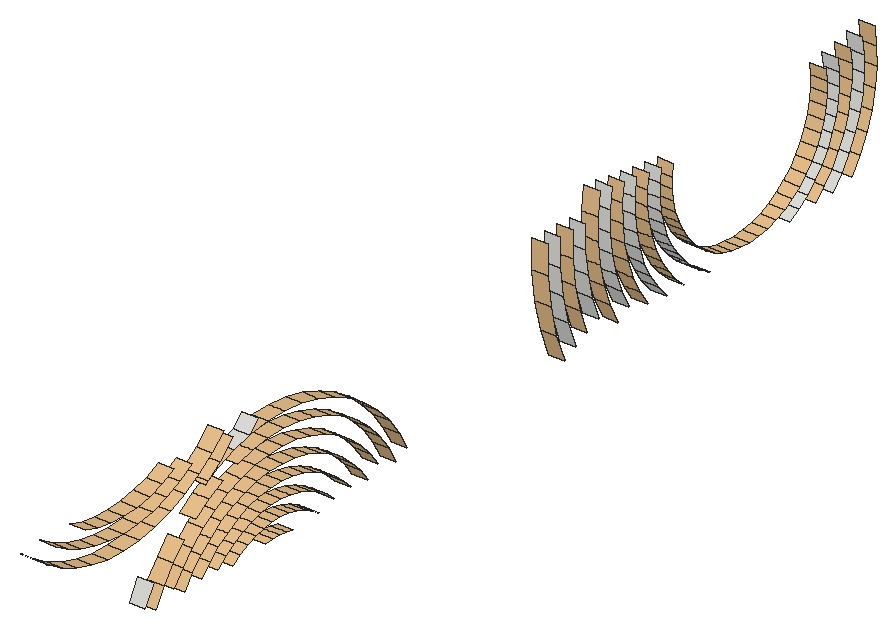
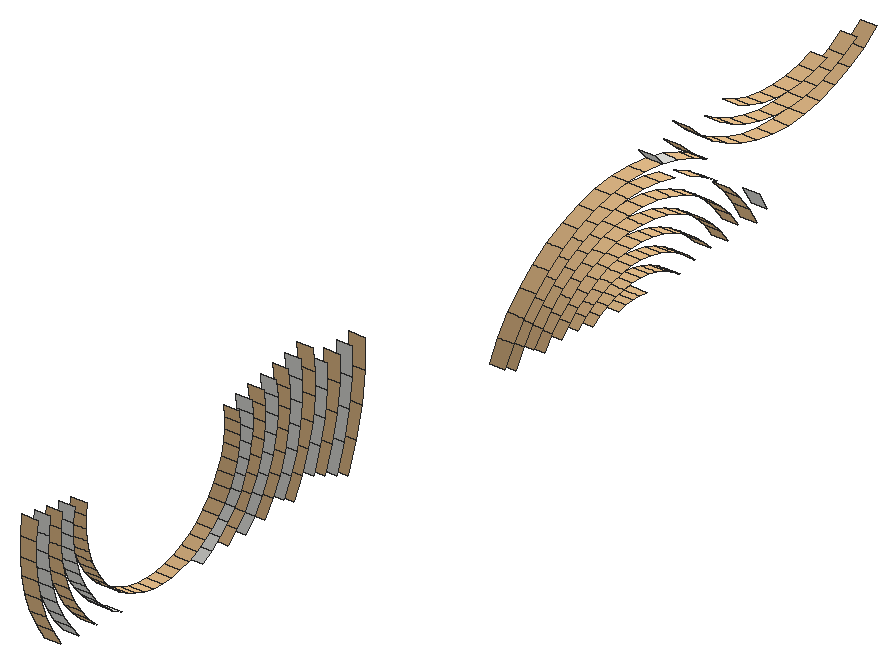
# SketchUp Ruby script. Lengths in inches.
U = 1.inch
M = Sketchup.active_model
def pt(a) = Geom::Point3d.new(a.map { |v| v * U })
def face(e, loops, mat)
  f = e.add_face(loops[0].map { |a| pt(a) })
  loops[1..].each { |l| e.add_face(l.map { |a| pt(a) }).erase! }
  f.material = f.back_material = mat if mat
  f
end
# faces: each face lists its corners as indices into pts; further lists are holes
def faces(e, pts, list, mat = nil) = list.each { |f| face(e, (f[0].is_a?(Array) ? f : [f]).map { |l| l.map { |i| pts[i] } }, mat) }
# xy, xz, yz: faces in a plane at the given z, y or x. An outline is a flat list of corners, or four numbers for a rectangle; further outlines are holes
def ring(l) = l.size == 4 ? [[l[0], l[1]], [l[2], l[1]], [l[2], l[3]], [l[0], l[3]]] : l.each_slice(2).to_a
def flat(e, list, mat, &to3) = list.each { |f| face(e, (f[0].is_a?(Array) ? f : [f]).map { |l| ring(l).map { |u, v| to3.(u, v) } }, mat) }
def xy(e, z, list, mat = nil) = flat(e, list, mat) { |x, y| [x, y, z] }
def xz(e, y, list, mat = nil) = flat(e, list, mat) { |x, z| [x, y, z] }
def yz(e, x, list, mat = nil) = flat(e, list, mat) { |y, z| [x, y, z] }
def lines(e, pts, list) = list.each { |a, b| e.add_line(pt(pts[a]), pt(pts[b])) }
# prism: a flat outline (further loops are holes) pulled along v
def prism(e, loops, v, mat = nil)
  f = face(e, loops, mat); d = Geom::Vector3d.new(v.map { |x| x * U })
  f.pushpull(f.normal.samedirection?(d) ? d.length : -d.length)
end
def box(e, o, s, mat = nil) = prism(e, [[o, [o[0] + s[0], o[1], o[2]], [o[0] + s[0], o[1] + s[1], o[2]], [o[0], o[1] + s[1], o[2]]]], [0, 0, s[2]], mat)
def at(x, y, z, deg = 0) = Geom::Transformation.translation(pt([x, y, z])) * Geom::Transformation.rotation(ORIGIN, Z_AXIS, deg.degrees)
def axes(o, x, y, z) = Geom::Transformation.new([*x, 0, *y, 0, *z, 0, *pt(o).to_a, 1])
def part(name) = M.definitions.add(name)
# library, detail: a bought-in or finely detailed component or shape, given as its bounding box
def library(name, o, s) = part(name).tap { |d| box(d.entities, o, s) }
def detail(e, o, s) = box(e.add_group.entities, o, s)
def put(e, d, t, mat = nil) = e.add_instance(d, t).tap { |i| i.material = mat if mat }
def group(e, t, mat = nil) = e.add_group.tap { |g| g.transformation = t; g.material = mat if mat }.entities
root = M.entities
M.materials.add("images").color = [235, 194, 141]
xy(root,18.6875,[[183.82,93.83,185.82,94.95]],"images")
xy(root,20.69,[[183.82,93.71,185.82,95.07]],"images")
xy(root,22.68,[[183.82,93.6,185.82,95.18]],"images")
xy(root,24.68,[[183.82,93.48,185.82,95.3]],"images")
xy(root,26.68,[[183.82,93.36,185.82,95.41]],"images")
xy(root,28.67,[[183.82,93.25,185.82,95.53]],"images")
xy(root,30.67,[[183.82,93.13,185.82,95.65]],"images")
xy(root,32.61,[[183.82,93.02,185.82,95.76]],"images")
xz(root,182.85,[[183.82,30.9375,185.82,32.39]],"images")
p = [[183.82,96.0625,18.56],[183.82,97.15,18.3],[185.82,97.15,18.3],[185.82,96.0625,18.56],[183.82,88.58,19.15],[183.82,87.45,18.4],
  [185.82,87.45,18.4],[185.82,88.58,19.15],[183.82,101.33,18.4],[183.82,100.2,19.15],[185.82,100.2,19.15],[185.82,101.33,18.4],
  [183.82,92.72,18.56],[183.82,93.83,18.6875],[185.82,93.83,18.6875],[185.82,92.72,18.56],[183.82,94.95,18.6875],[185.82,94.95,18.6875],
  [183.82,139.41,22.1],[183.82,140.73,18.57],[185.82,140.73,18.57],[185.82,139.41,22.1],[183.82,164.03,18.65],[183.82,162.57,19.48],
  [185.82,162.57,19.48],[185.82,164.03,18.65],[183.82,178.4375,19.57],[183.82,176.99,18.73],[185.82,176.99,18.73],[185.82,178.4375,19.57],
  [183.82,75.06,18.79],[183.82,76.32,20.96],[185.82,76.32,20.96],[185.82,75.06,18.79],[183.82,79.66,18.77],[183.82,80.89,20.41],
  [185.82,80.89,20.41],[185.82,79.66,18.77],[183.82,107.89,20.41],[183.82,109.12,18.77],[185.82,109.12,18.77],[185.82,107.89,20.41],
  [183.82,112.46,20.96],[183.82,113.71,18.79],[185.82,113.71,18.79],[185.82,112.46,20.96],[183.82,157.1,18.86],[183.82,155.71,20.49],
  [185.82,155.71,20.49],[185.82,157.1,18.86],[183.82,158.54,20.24],[183.82,159.94,18.94],[185.82,159.94,18.94],[185.82,158.54,20.24],
  [183.82,85.04,18.99],[183.82,86.25,20.01],[185.82,86.25,20.01],[185.82,85.04,18.99],[183.82,102.53,20.01],[183.82,103.74,18.99],
  [185.82,103.74,18.99],[185.82,102.53,20.01],[183.82,185.29,20.67],[183.82,183.92,19.02],[185.82,183.92,19.02],[185.82,185.29,20.67],
  [183.82,83.67,20.45],[183.82,82.42,19.125],[185.82,82.42,19.125],[185.82,83.67,20.45],[183.82,89.79,19.75],[185.82,89.79,19.75],
  [183.82,98.99,19.75],[185.82,98.99,19.75],[183.82,106.36,19.125],[183.82,105.11,20.45],[185.82,105.11,20.45],[185.82,106.36,19.125],
  [183.82,181.07,19.06],[183.82,182.46,20.38],[185.82,182.46,20.38],[185.82,181.07,19.06],[183.82,148.05,21.78],[183.82,149.34,19.25],
  [185.82,149.34,19.25],[185.82,148.05,21.78],[183.82,167.64,19.47],[183.82,169.0625,19.23],[185.82,169.0625,19.23],[185.82,167.64,19.47],
  [183.82,170.51,19.15],[185.82,170.51,19.15],[183.82,171.95,19.24],[185.82,171.95,19.24],[183.82,173.375,19.5],[185.82,173.375,19.5],
  [183.82,152.8,21.27],[183.82,154.11,19.29],[185.82,154.11,19.29],[185.82,152.8,21.27],[183.82,142.56,19.37],[183.82,141.33,22.6875],
  [185.82,141.33,22.6875],[185.82,142.56,19.37],[183.82,161.22,20.47],[185.82,161.22,20.47],[183.82,166.25,19.875],[185.82,166.25,19.875],
  [183.82,174.76,19.93],[185.82,174.76,19.93],[183.82,186.9,19.48],[183.82,188.19,21.48],[185.82,188.19,21.48],[185.82,186.9,19.48],
  [183.82,179.78,20.58],[185.82,179.78,20.58],[183.82,74.7,22.03],[183.82,73.33,19.66],[185.82,73.33,19.66],[185.82,74.7,22.03],
  [183.82,115.45,19.66],[183.82,114.08,22.03],[185.82,114.08,22.03],[185.82,115.45,19.66],[183.82,91.06,20.22],[185.82,91.06,20.22],
  [183.82,97.72,20.22],[185.82,97.72,20.22],[183.82,79.36,21.69],[183.82,77.99,19.86],[185.82,77.99,19.86],[185.82,79.36,21.69],
  [183.82,110.79,19.86],[183.82,109.42,21.69],[185.82,109.42,21.69],[185.82,110.79,19.86],[183.82,164.92,20.44],[185.82,164.92,20.44],
  [183.82,176.08,20.51],[185.82,176.08,20.51],[183.82,87.58,20.88],[185.82,87.58,20.88],[183.82,101.2,20.88],[185.82,101.2,20.88],
  [183.82,92.37,20.53],[185.82,92.37,20.53],[183.82,96.41,20.53],[185.82,96.41,20.53],[183.82,143.24,23.27],[183.82,144.39,20.17],
  [185.82,144.39,20.17],[185.82,143.24,23.27],[183.82,157.31,21.7],[185.82,157.31,21.7],[183.82,151.07,20.26],[183.82,149.88,22.58],
  [185.82,149.88,22.58],[185.82,151.07,20.26],[183.82,82.29,21.9],[185.82,82.29,21.9],[183.82,85.06,21.61],[185.82,85.06,21.61],
  [183.82,103.72,21.61],[185.82,103.72,21.61],[183.82,106.48,21.9],[185.82,106.48,21.9],[183.82,163.66,21.16],[185.82,163.66,21.16],
  [183.82,183.68,21.85],[185.82,183.68,21.85],[183.82,93.71,20.69],[185.82,93.71,20.69],[183.82,95.07,20.69],[185.82,95.07,20.69],
  [183.82,154.52,22.28],[185.82,154.52,22.28],[183.82,159.99,21.62],[185.82,159.99,21.62],[183.82,177.33,21.24],[185.82,177.33,21.24],
  [183.82,180.99,21.74],[185.82,180.99,21.74],[183.82,186.46,22.46],[185.82,186.46,22.46],[183.82,88.99,21.59],[185.82,88.99,21.59],
  [183.82,99.79,21.59],[185.82,99.79,21.59],[183.82,77.82,22.98],[185.82,77.82,22.98],[183.82,110.96,22.98],[185.82,110.96,22.98],
  [183.82,146.22,20.97],[183.82,145.15,23.86],[185.82,145.15,23.86],[185.82,146.22,20.97],[183.82,162.5,22.01],[185.82,162.5,22.01],
  [183.82,178.49,22.11],[185.82,178.49,22.11],[183.82,151.72,23.38],[185.82,151.72,23.38],[183.82,189.25,23.61],[185.82,189.25,23.61],
  [183.82,86.58,22.61],[185.82,86.58,22.61],[183.82,90.48,22.13],[185.82,90.48,22.13],[183.82,98.3,22.13],[185.82,98.3,22.13],
  [183.82,102.2,22.61],[185.82,102.2,22.61],[183.82,158.9,22.9],[185.82,158.9,22.9],[183.82,80.92,23.35],[185.82,80.92,23.35],
  [183.82,107.86,23.35],[185.82,107.86,23.35],[183.82,156.25,23.29],[185.82,156.25,23.29],[183.82,182.07,23.04],[185.82,182.07,23.04],
  [183.82,147.07,24.44],[185.82,147.07,24.44],[183.82,83.86,23.22],[185.82,83.86,23.22],[183.82,104.91,23.22],[185.82,104.91,23.22],
  [183.82,184.72,23.45],[185.82,184.72,23.45],[183.82,112.44,24.23],[185.82,112.44,24.23],[183.82,161.4375,23],[185.82,161.4375,23],
  [183.82,92.02,22.5],[185.82,92.02,22.5],[183.82,96.76,22.5],[185.82,96.76,22.5],[183.82,138.52,25.77],[185.82,138.52,25.77],
  [183.82,179.53,23.11],[185.82,179.53,23.11],[183.82,153.55,24.1875],[185.82,153.55,24.1875],[183.82,93.6,22.68],[185.82,93.6,22.68],
  [183.82,95.18,22.68],[185.82,95.18,22.68],[183.82,187.41,24.39],[185.82,187.41,24.39],[183.82,88.2,23.43],[185.82,88.2,23.43],
  [183.82,100.58,23.43],[185.82,100.58,23.43],[183.82,148.98,25.03],[185.82,148.98,25.03],[183.82,140.49,26.125],[185.82,140.49,26.125],
  [183.82,157.97,24.3],[185.82,157.97,24.3],[183.82,79.55,24.81],[185.82,79.55,24.81],[183.82,109.23,24.81],[185.82,109.23,24.81],
  [183.82,160.5,24.1],[185.82,160.5,24.1],[183.82,182.98,24.44],[185.82,182.98,24.44],[183.82,180.45,24.22],[185.82,180.45,24.22],
  [183.82,85.58,24.34],[185.82,85.58,24.34],[183.82,103.2,24.34],[185.82,103.2,24.34],[183.82,142.46,26.49],[185.82,142.46,26.49],
  [183.82,155.38,24.99],[185.82,155.38,24.99],[183.82,82.67,24.82],[185.82,82.67,24.82],[183.82,89.91,24.05],[185.82,89.91,24.05],
  [183.82,98.87,24.05],[185.82,98.87,24.05],[183.82,106.11,24.82],[185.82,106.11,24.82],[183.82,150.89,25.61],[185.82,150.89,25.61],
  [183.82,185.57,25.17],[185.82,185.57,25.17],[183.82,190.05,25.84],[185.82,190.05,25.84],[183.82,144.43,26.84],[185.82,144.43,26.84],
  [183.82,91.68,24.47],[185.82,91.68,24.47],[183.82,97.1,24.47],[185.82,97.1,24.47],[183.82,159.7,25.31],[185.82,159.7,25.31],
  [183.82,110.5625,26.22],[185.82,110.5625,26.22],[183.82,152.8,26.2],[185.82,152.8,26.2],[183.82,181.24,25.43],[185.82,181.24,25.43],
  [183.82,87.41,25.26],[185.82,87.41,25.26],[183.82,101.37,25.26],[185.82,101.37,25.26],[183.82,157.21,25.79],[185.82,157.21,25.79],
  [183.82,146.39,27.2],[185.82,146.39,27.2],[183.82,183.72,25.95],[185.82,183.72,25.95],[183.82,188.13,26.41],[185.82,188.13,26.41],
  [183.82,93.48,24.68],[185.82,93.48,24.68],[183.82,95.3,24.68],[185.82,95.3,24.68],[183.82,84.58,26.08],[185.82,84.58,26.08],
  [183.82,104.2,26.08],[185.82,104.2,26.08],[183.82,107.3,26.43],[185.82,107.3,26.43],[183.82,148.36,27.5625],[185.82,148.36,27.5625],
  [183.82,154.72,26.78],[185.82,154.72,26.78],[183.82,186.21,26.97],[185.82,186.21,26.97],[183.82,89.33,25.96],[185.82,89.33,25.96],
  [183.82,99.44,25.96],[185.82,99.44,25.96],[183.82,159.04,26.6],[185.82,159.04,26.6],[183.82,181.88,26.73],[185.82,181.88,26.73],
  [183.82,150.33,27.92],[185.82,150.33,27.92],[183.82,138.0625,29.51],[185.82,138.0625,29.51],[183.82,156.63,27.37],[185.82,156.63,27.37],
  [183.82,190.58,28.16],[185.82,190.58,28.16],[183.82,184.29,27.53],[185.82,184.29,27.53],[183.82,91.33,26.4375],[185.82,91.33,26.4375],
  [183.82,97.45,26.4375],[185.82,97.45,26.4375],[183.82,86.62,27.1],[185.82,86.62,27.1],[183.82,102.16,27.1],[185.82,102.16,27.1],
  [183.82,140.06,29.64],[185.82,140.06,29.64],[183.82,108.46,27.98],[185.82,108.46,27.98],[183.82,152.3,28.28],[185.82,152.3,28.28],
  [183.82,81.48,26.43],[183.82,83.58,27.81],[185.82,83.58,27.81],[185.82,81.48,26.43],[183.82,93.36,26.68],[185.82,93.36,26.68],
  [183.82,95.41,26.68],[185.82,95.41,26.68],[183.82,105.2,27.81],[185.82,105.2,27.81],[183.82,188.61,28.49],[185.82,188.61,28.49],
  [183.82,142.06,29.77],[185.82,142.06,29.77],[183.82,158.54,27.95],[185.82,158.54,27.95],[183.82,182.37,28.09],[185.82,182.37,28.09],
  [183.82,144.05,29.9],[185.82,144.05,29.9],[183.82,154.26,28.64],[185.82,154.26,28.64],[183.82,186.64,28.83],[185.82,186.64,28.83],
  [183.82,88.76,27.88],[185.82,88.76,27.88],[183.82,100.02,27.88],[185.82,100.02,27.88],[183.82,146.05,30.02],[185.82,146.05,30.02],
  [183.82,156.23,29],[185.82,156.23,29],[183.82,184.67,29.17],[185.82,184.67,29.17],[183.82,148.04,30.15],[185.82,148.04,30.15],
  [183.82,67.36,27.94],[183.82,69.91,27.78],[185.82,69.91,27.78],[185.82,67.36,27.94],[183.82,72.47,27.92],[185.82,72.47,27.92],
  [183.82,85.82,28.9375],[185.82,85.82,28.9375],[183.82,102.96,28.9375],[185.82,102.96,28.9375],[183.82,64.84,28.4],[185.82,64.84,28.4],
  [183.82,74.99,28.35],[185.82,74.99,28.35],[183.82,90.98,28.41],[185.82,90.98,28.41],[183.82,97.8,28.41],[185.82,97.8,28.41],
  [183.82,150.04,30.28],[185.82,150.04,30.28],[183.82,106.17,29.49],[185.82,106.17,29.49],[183.82,158.2,29.36],[185.82,158.2,29.36],
  [183.82,182.7,29.5],[185.82,182.7,29.5],[183.82,190.84,30.52],[185.82,190.84,30.52],[183.82,152.03,30.41],[185.82,152.03,30.41],
  [183.82,62.39,29.15],[185.82,62.39,29.15],[183.82,77.44,29.07],[185.82,77.44,29.07],[183.82,93.25,28.67],[185.82,93.25,28.67],
  [183.82,95.53,28.67],[185.82,95.53,28.67],[183.82,188.85,30.625],[185.82,188.85,30.625],[183.82,154.03,30.54],[185.82,154.03,30.54],
  [183.82,186.85,30.73],[185.82,186.85,30.73],[183.82,100.59,29.8],[185.82,100.59,29.8],[183.82,156.03,30.66],[185.82,156.03,30.66],
  [183.82,60.05,30.17],[185.82,60.05,30.17],[183.82,79.8,30.07],[185.82,79.8,30.07],[183.82,184.85,30.83],[185.82,184.85,30.83],
  [183.82,158.02,30.79],[185.82,158.02,30.79],[183.82,103.72,30.72],[185.82,103.72,30.72],[183.82,138.04,33.28],[185.82,138.04,33.28],
  [183.82,182.85,30.9375],[185.82,182.85,30.9375],[183.82,140.04,33.18],[185.82,140.04,33.18],[183.82,83.42,29.9],[183.82,83.11,29.67],
  [185.82,83.11,29.67],[185.82,83.42,29.9],[183.82,69.92,29.78],[183.82,67.6,29.93],[185.82,67.6,29.93],[185.82,69.92,29.78],
  [183.82,72.24,29.91],[185.82,72.24,29.91],[183.82,88.1875,29.8],[183.82,90.63,30.375],[185.82,90.63,30.375],[185.82,88.1875,29.8],
  [183.82,98.14,30.375],[185.82,98.14,30.375],[183.82,142.04,33.08],[185.82,142.04,33.08],[183.82,65.3125,30.35],[185.82,65.3125,30.35],
  [183.82,74.54,30.3],[185.82,74.54,30.3],[183.82,85.06,30.72],[185.82,85.06,30.72],[183.82,85.36,31.32],[185.82,85.36,31.32],
  [183.82,144.03,32.97],[185.82,144.03,32.97],[183.82,146.03,32.87],[185.82,146.03,32.87],[183.82,82.02,31.34],[185.82,82.02,31.34],
  [183.82,57.84,31.46],[185.82,57.84,31.46],[183.82,148.03,32.76],[185.82,148.03,32.76],[183.82,63.09,31.02],[185.82,63.09,31.02],
  [183.82,76.77,30.96],[185.82,76.77,30.96],[183.82,150.02,32.66],[185.82,150.02,32.66],[183.82,93.13,30.67],[185.82,93.13,30.67],
  [183.82,95.65,30.67],[185.82,95.65,30.67],[183.82,152.02,32.55],[185.82,152.02,32.55],[183.82,154.02,32.45],[185.82,154.02,32.45],
  [183.82,190.83,32.9],[185.82,190.83,32.9],[183.82,188.83,32.77],[185.82,188.83,32.77],[183.82,87.63,31.65],[185.82,87.63,31.65],
  [183.82,101.15,31.65],[185.82,101.15,31.65],[183.82,156.02,32.34],[185.82,156.02,32.34],[183.82,186.84,32.64],[185.82,186.84,32.64],
  [183.82,158.01,32.24],[185.82,158.01,32.24],[183.82,184.84,32.51],[185.82,184.84,32.51],[183.82,60.96,31.95],[185.82,60.96,31.95],
  [183.82,78.91,31.87],[185.82,78.91,31.87],[183.82,84.08,32.86],[185.82,84.08,32.86],[183.82,87.4,33.23],[185.82,87.4,33.23],
  [183.82,55.8,33],[185.82,55.8,33],[183.82,90.15,32.25],[185.82,90.15,32.25],[183.82,98.48,32.29],[185.82,98.48,32.29],
  [183.82,67.84,31.92],[183.82,69.93,31.78],[185.82,69.93,31.78],[185.82,67.84,31.92],[183.82,72.02,31.89],[185.82,72.02,31.89],
  [183.82,65.78,32.29],[185.82,65.78,32.29],[183.82,74.09,32.25],[185.82,74.09,32.25],[183.82,80.93,33.02],[185.82,80.93,33.02],
  [183.82,58.95,33.13],[185.82,58.95,33.13],[183.82,76.09,32.84],[185.82,76.09,32.84],[183.82,158.17,33.68],[185.82,158.17,33.68],
  [183.82,63.78,32.9],[185.82,63.78,32.9],[183.82,90.3,32.29],[185.82,90.3,32.29],[183.82,91.39,33.71],[185.82,91.39,33.71],
  [183.82,93.02,32.61],[185.82,93.02,32.61],[183.82,95.76,32.61],[185.82,95.76,32.61],[183.82,156.2,34.01],[185.82,156.2,34.01],
  [183.82,154.23,34.35],[185.82,154.23,34.35],[183.82,182.85,32.39],[183.82,182.67,33.82],[185.82,182.67,33.82],[185.82,182.85,32.39],
  [183.82,184.64,34.18],[185.82,184.64,34.18],[183.82,152.26,34.68],[185.82,152.26,34.68],[183.82,186.6,34.54],[185.82,186.6,34.54],
  [183.82,150.29,35.02],[185.82,150.29,35.02],[183.82,78.02,33.66],[185.82,78.02,33.66],[183.82,148.32,35.35],[185.82,148.32,35.35],
  [183.82,188.57,34.9],[185.82,188.57,34.9],[183.82,85.95,34.61],[185.82,85.95,34.61],[183.82,146.34,35.69],[185.82,146.34,35.69],
  [183.82,190.54,35.26],[185.82,190.54,35.26]]
faces(root,p,[[0,1,2,3],[4,5,6,7],[8,9,10,11],[12,13,14,15],[16,0,3,17],[18,19,20,21],[30,31,32,33],[34,35,36,37],
  [38,39,40,41],[42,43,44,45],[50,51,52,53],[54,55,56,57],[58,59,60,61],[66,67,68,69],[70,4,7,71],[9,72,73,10],
  [74,75,76,77],[78,79,80,81],[82,83,84,85],[86,87,88,89],[87,90,91,88],[90,92,93,91],[92,94,95,93],[96,97,98,99],
  [106,86,89,107],[94,108,109,95],[110,111,112,113],[120,121,122,123],[124,70,71,125],[72,126,127,73],[128,129,130,131],[132,133,134,135],
  [136,106,107,137],[108,138,139,109],[55,140,141,56],[142,58,61,143],[144,124,125,145],[126,146,147,127],[148,149,150,151],[152,50,53,153],
  [35,158,159,36],[160,66,69,161],[75,162,163,76],[164,38,41,165],[166,136,137,167],[79,168,169,80],[170,144,145,171],[146,172,173,147],
  [138,178,179,139],[140,184,185,141],[186,142,143,187],[31,188,189,32],[190,42,45,191],[196,166,167,197],[178,198,199,179],[200,96,99,201],
  [111,202,203,112],[204,160,161,205],[184,206,207,185],[208,186,187,209],[162,210,211,163],[214,128,131,215],[133,216,217,134],[218,152,153,219],
  [222,82,85,223],[158,224,225,159],[226,164,165,227],[168,228,229,169],[121,230,231,122],[232,196,197,233],[206,234,235,207],[236,208,209,237],
  [238,18,21,239],[198,240,241,199],[234,244,245,235],[246,236,237,247],[250,204,205,251],[210,252,253,211],[188,260,261,189],[262,190,191,263],
  [264,232,233,265],[240,268,269,241],[224,270,271,225],[272,226,227,273],[274,148,151,275],[276,218,219,277],[278,214,215,279],[280,250,251,281],
  [252,282,283,253],[216,284,285,217],[286,200,201,287],[228,288,289,229],[202,290,291,203],[294,280,281,295],[282,296,297,283],[298,264,265,299],
  [230,300,301,231],[268,304,305,269],[270,306,307,271],[308,272,273,309],[312,222,223,313],[318,294,295,319],[296,320,321,297],[322,278,279,323],
  [284,324,325,285],[326,262,263,327],[330,276,277,331],[288,332,333,289],[306,334,335,307],[336,308,309,337],[338,298,299,339],[304,340,341,305],
  [342,286,287,343],[344,238,239,345],[290,348,349,291],[334,352,353,335],[354,336,337,355],[356,322,323,357],[324,358,359,325],[300,362,363,301],
  [366,367,368,369],[352,370,371,353],[372,354,355,373],[374,326,327,375],[378,274,275,379],[380,338,339,381],[340,382,383,341],[386,330,331,387],
  [332,388,389,333],[390,356,357,391],[358,392,393,359],[394,312,313,395],[402,403,404,405],[403,406,407,404],[367,408,409,368],[410,374,375,411],
  [412,402,405,413],[406,414,415,407],[416,390,391,417],[392,418,419,393],[420,342,343,421],[362,422,423,363],[424,380,381,425],[382,426,427,383],
  [348,428,429,349],[432,412,413,433],[414,434,435,415],[436,416,417,437],[418,438,439,419],[442,386,387,443],[388,444,445,389],[446,410,411,447],
  [450,432,433,451],[434,452,453,435],[456,424,425,457],[422,458,459,423],[460,344,345,461],[426,462,463,427],[466,467,468,469],[470,471,472,473],
  [474,470,473,475],[476,477,478,479],[480,446,447,481],[482,378,379,483],[471,484,485,472],[486,474,475,487],[488,466,469,489],[490,466,469,491],
  [494,394,395,495],[452,496,497,453],[498,450,451,499],[484,502,503,485],[504,486,487,505],[506,420,421,507],[477,508,509,478],[510,480,481,511],
  [514,442,443,515],[428,516,517,429],[520,488,489,521],[458,522,523,459],[444,526,527,445],[528,456,457,529],[502,532,533,503],[534,504,505,535],
  [496,536,537,497],[538,490,491,539],[540,498,499,541],[522,544,545,523],[546,547,548,549],[547,550,551,548],[552,546,549,553],[550,554,555,551],
  [556,534,535,557],[532,558,559,533],[554,560,561,555],[562,528,529,563],[564,552,553,565],[566,542,543,567],[570,566,567,571],[544,572,573,545],
  [576,514,515,577],[578,579,580,581],[526,586,587,527],[588,506,507,589],[560,590,591,561],[536,596,597,537],[598,494,495,599],[516,600,601,517]],"images")
faces(root,p,[[22,23,24,25],[26,27,28,29],[46,47,48,49],[62,63,64,65],[100,101,102,103],[23,104,105,24],[114,26,29,115],[116,117,118,119],
  [154,155,156,157],[47,174,175,48],[104,176,177,105],[180,114,115,181],[182,62,65,183],[192,193,194,195],[176,212,213,177],[220,180,181,221],
  [174,242,243,175],[248,182,183,249],[155,254,255,156],[101,256,257,102],[212,258,259,213],[266,220,221,267],[193,292,293,194],[242,302,303,243],
  [258,310,311,259],[314,266,267,315],[316,248,249,317],[254,328,329,255],[310,346,347,311],[350,314,315,351],[256,360,361,257],[302,364,365,303],
  [376,316,317,377],[292,384,385,293],[346,396,397,347],[398,350,351,399],[328,400,401,329],[364,430,431,365],[440,376,377,441],[396,448,449,397],
  [454,398,399,455],[360,464,465,361],[384,492,493,385],[400,500,501,401],[430,512,513,431],[518,440,441,519],[448,524,525,449],[530,454,455,531],
  [542,520,521,543],[542,568,569,543],[524,574,575,525],[582,530,531,583],[512,584,585,513],[500,592,593,501],[594,518,519,595]])
